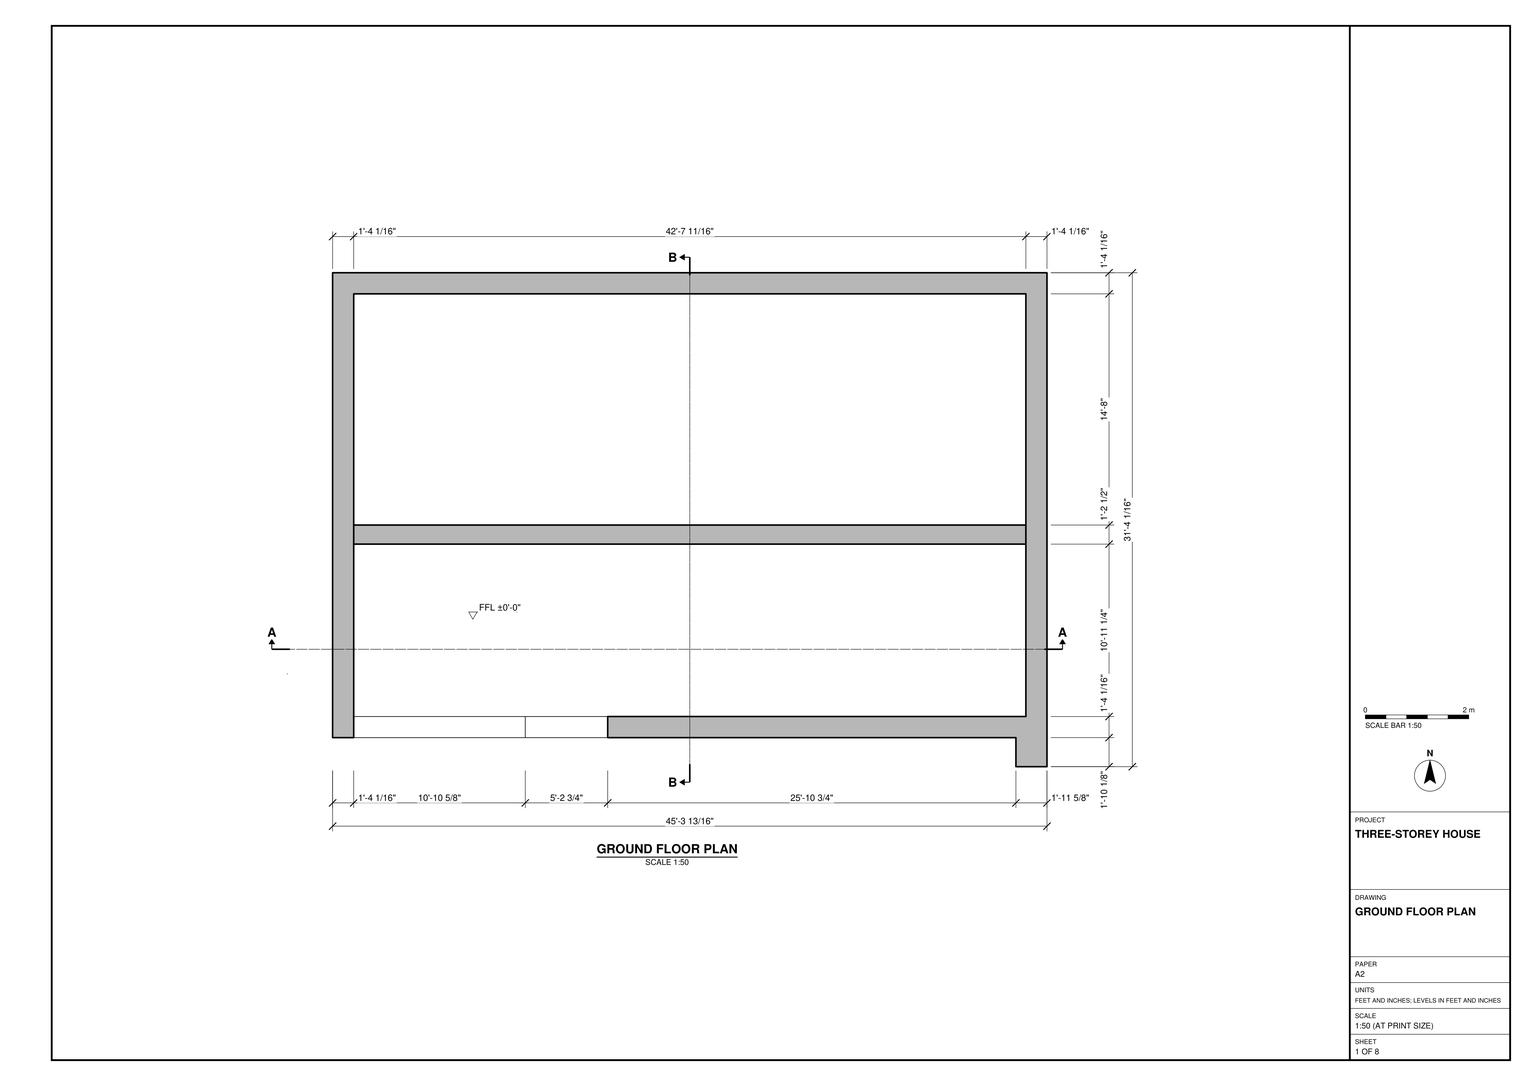
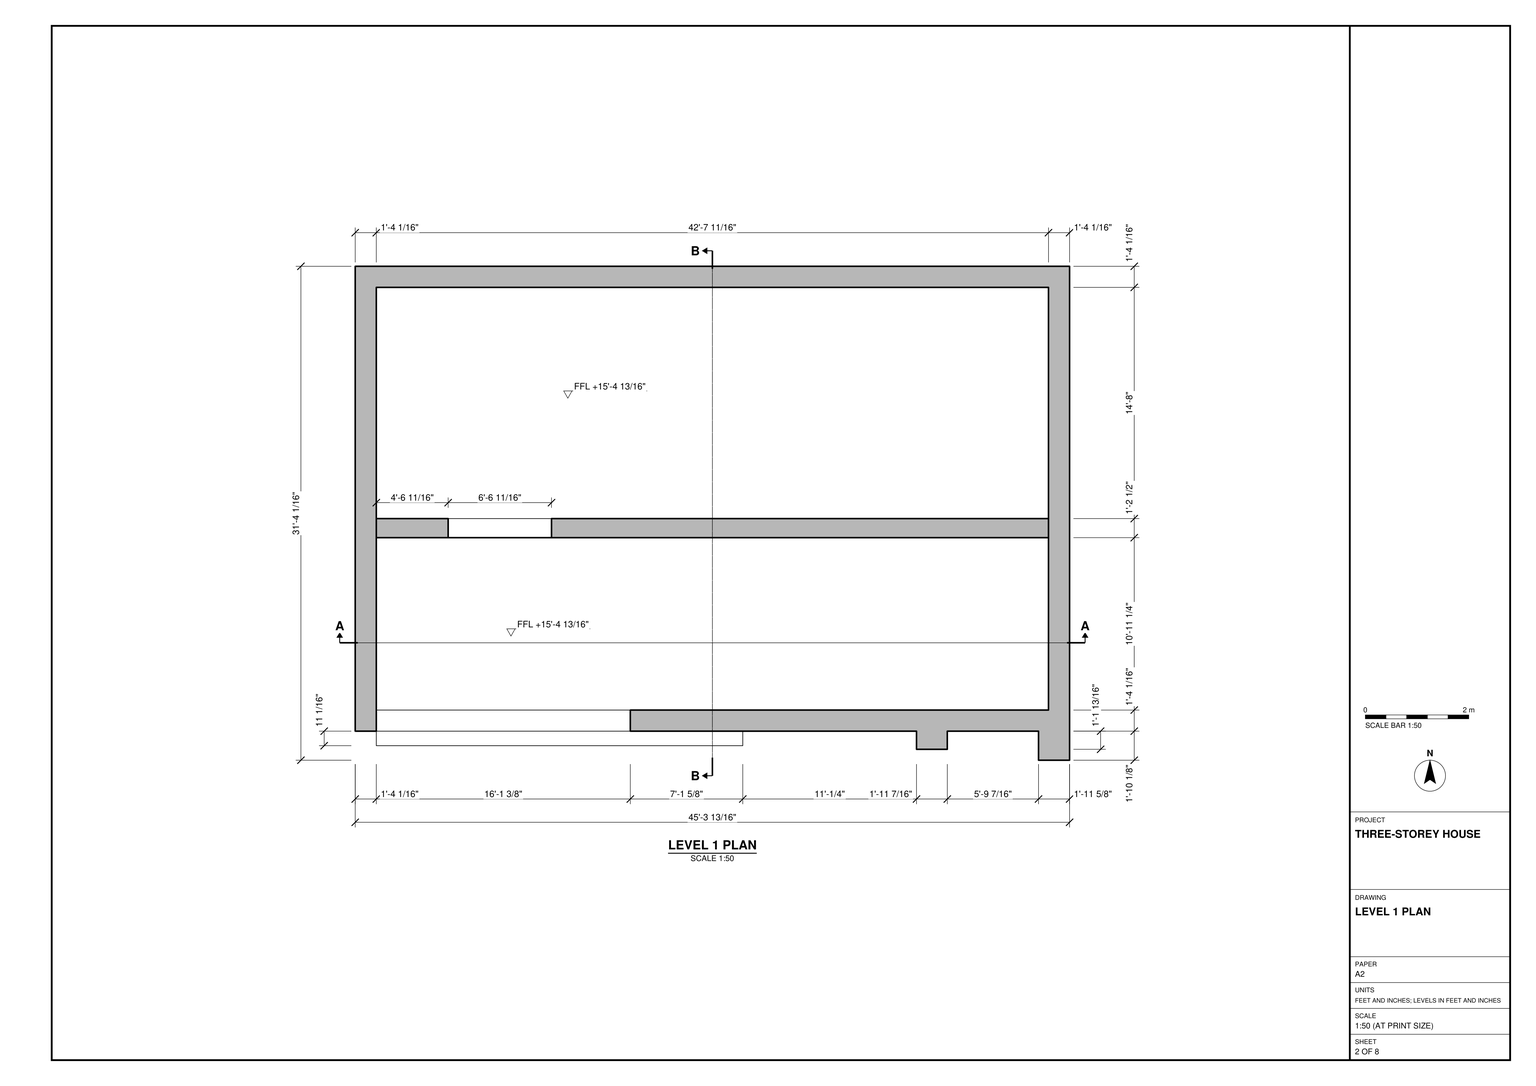
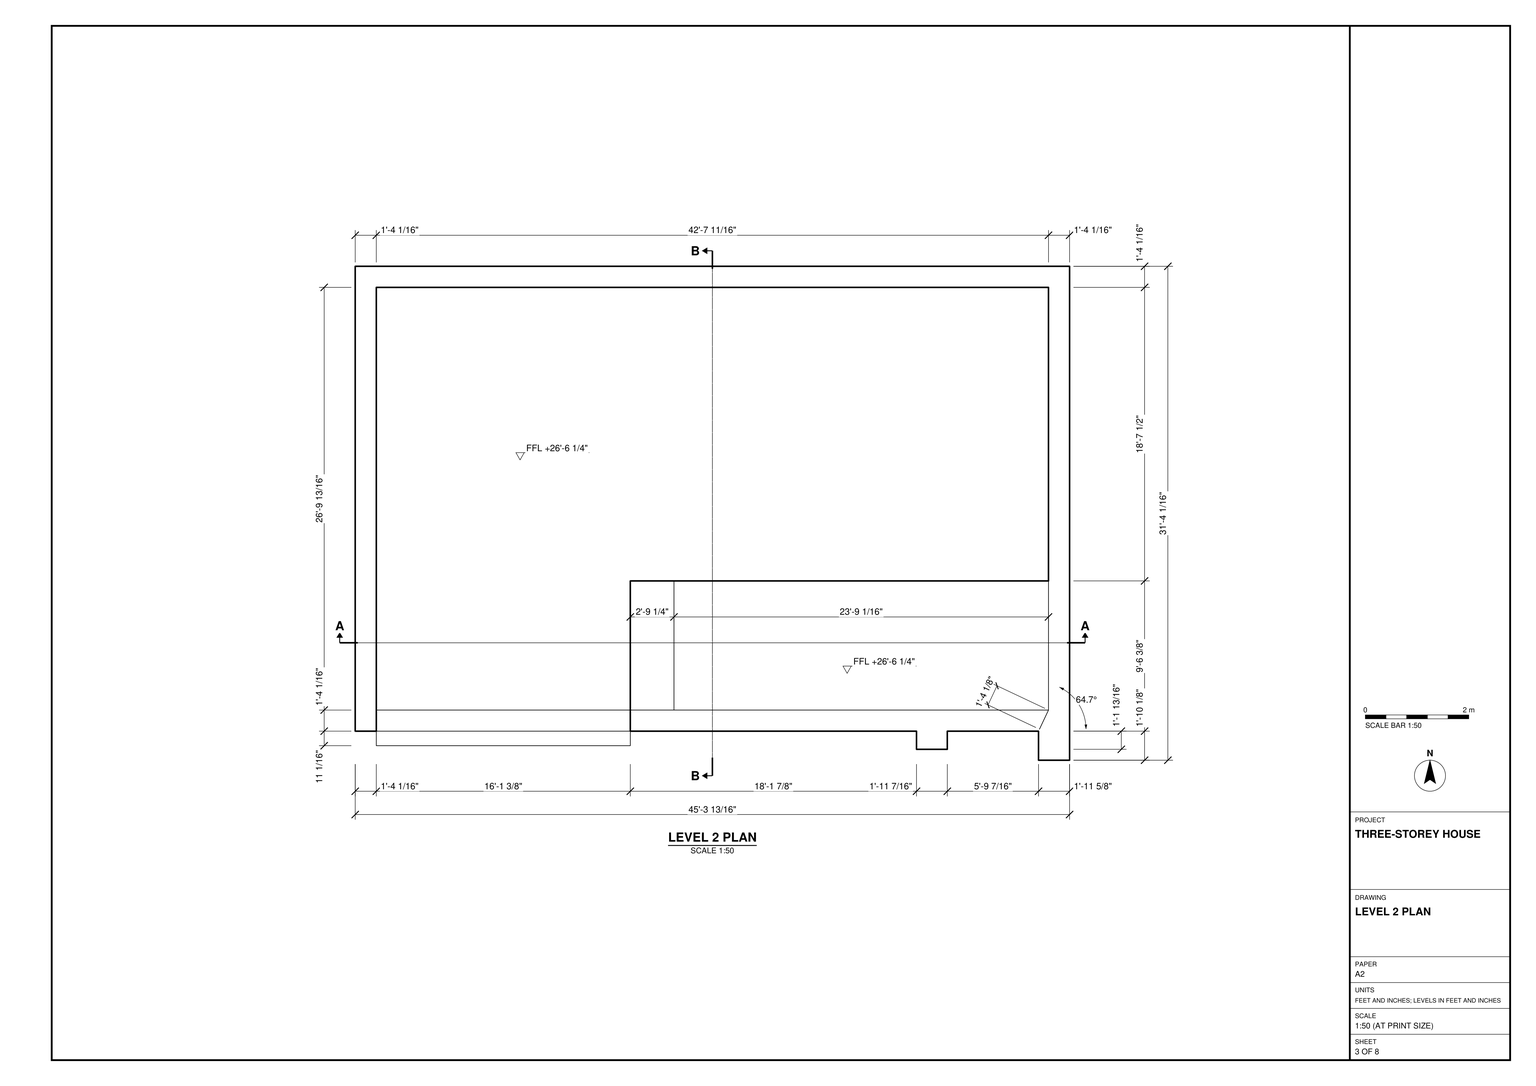
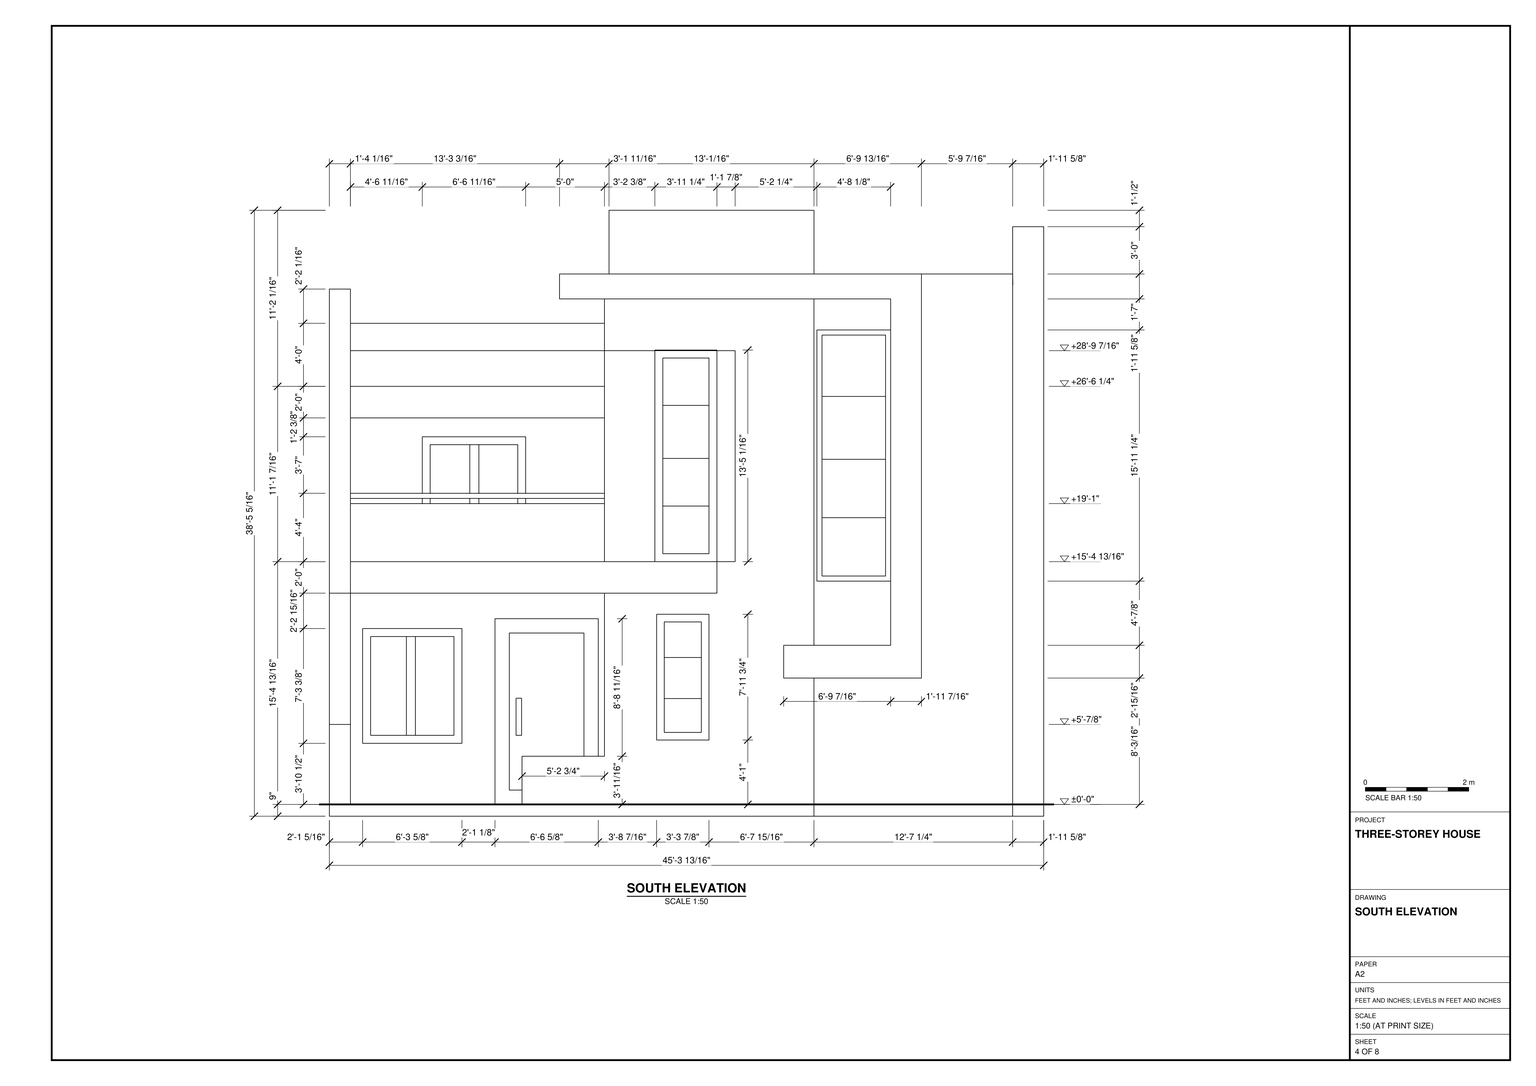
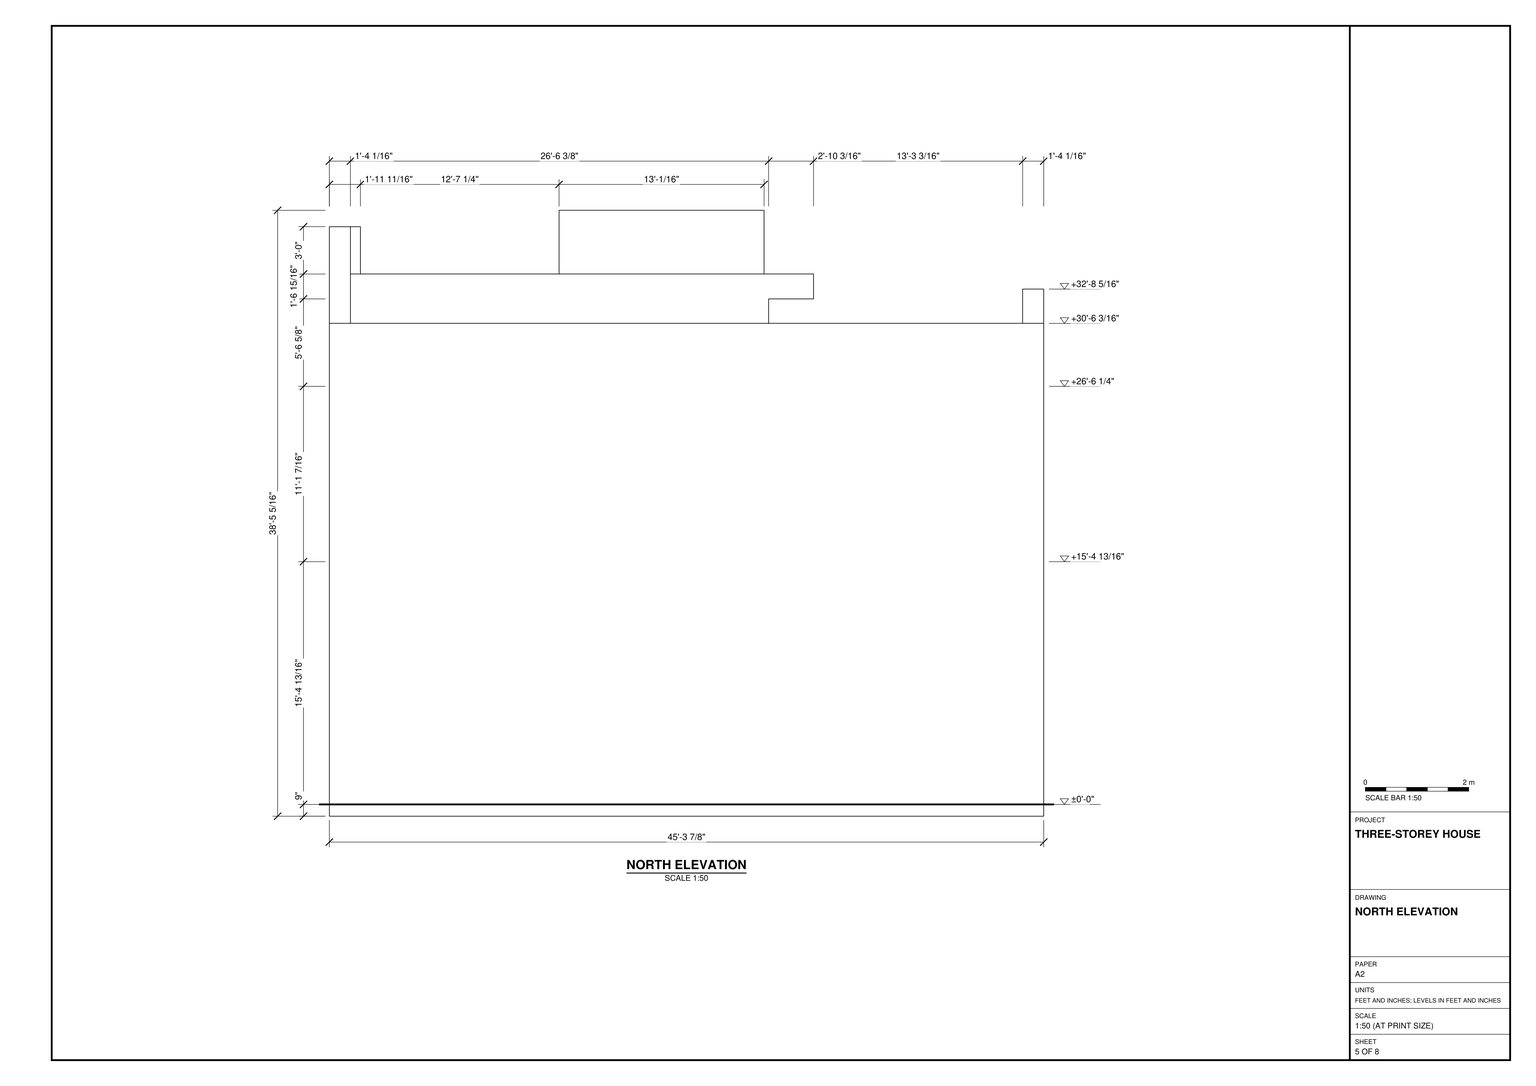
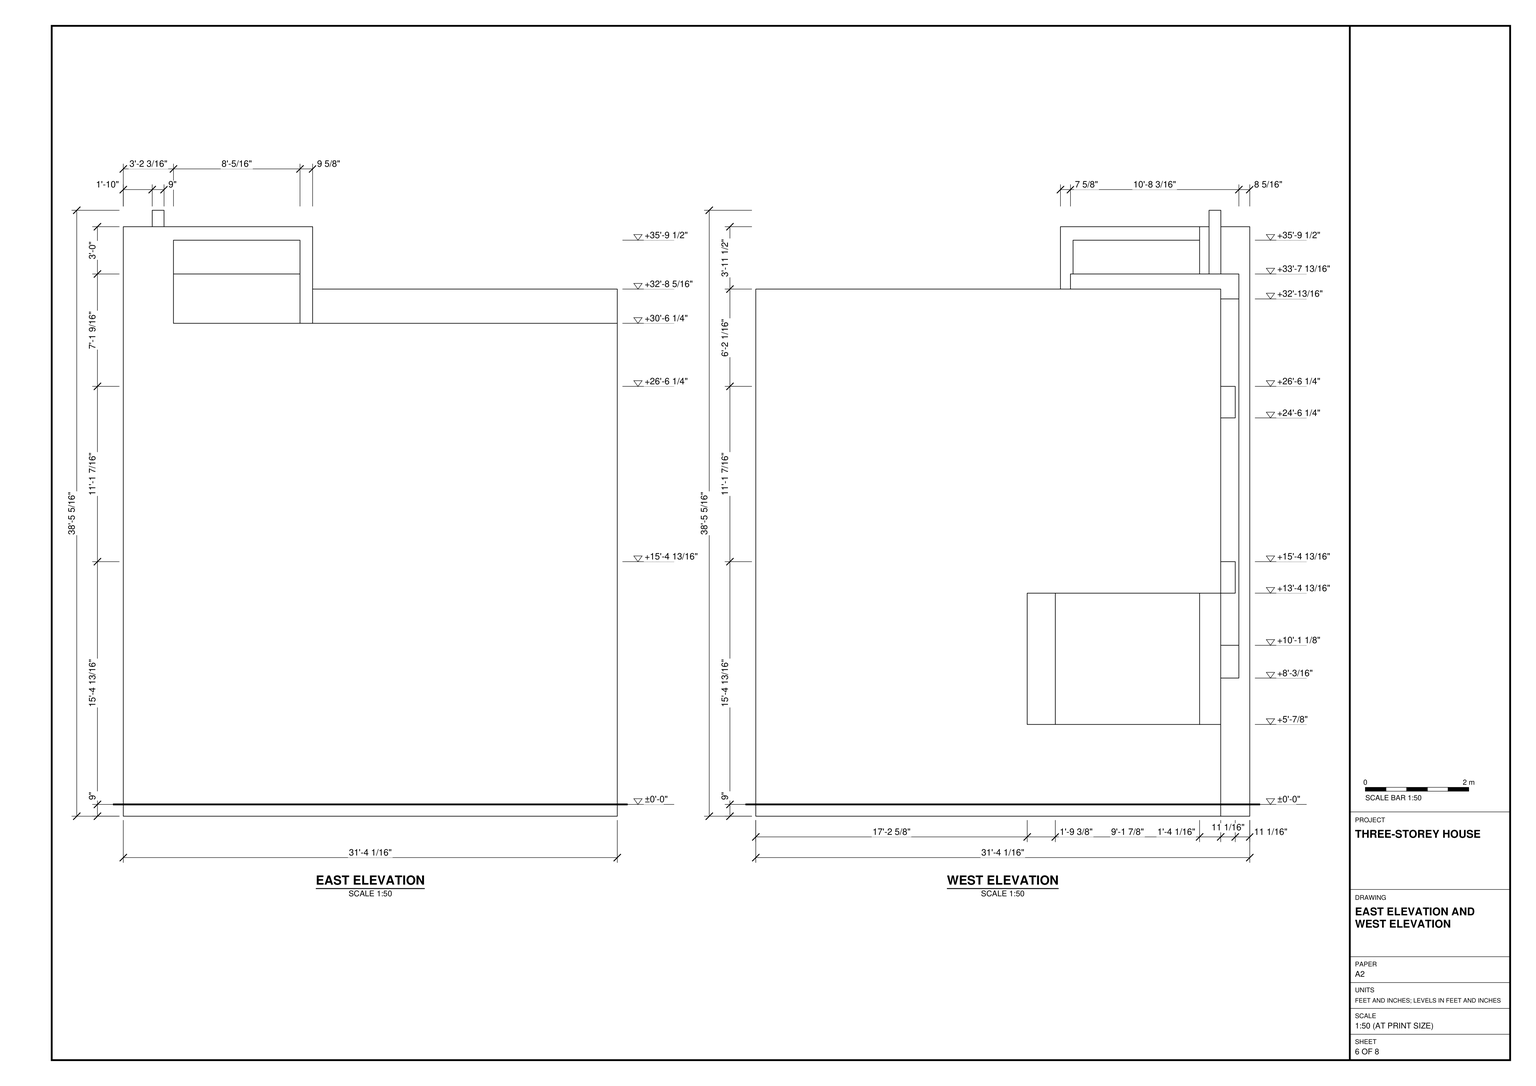
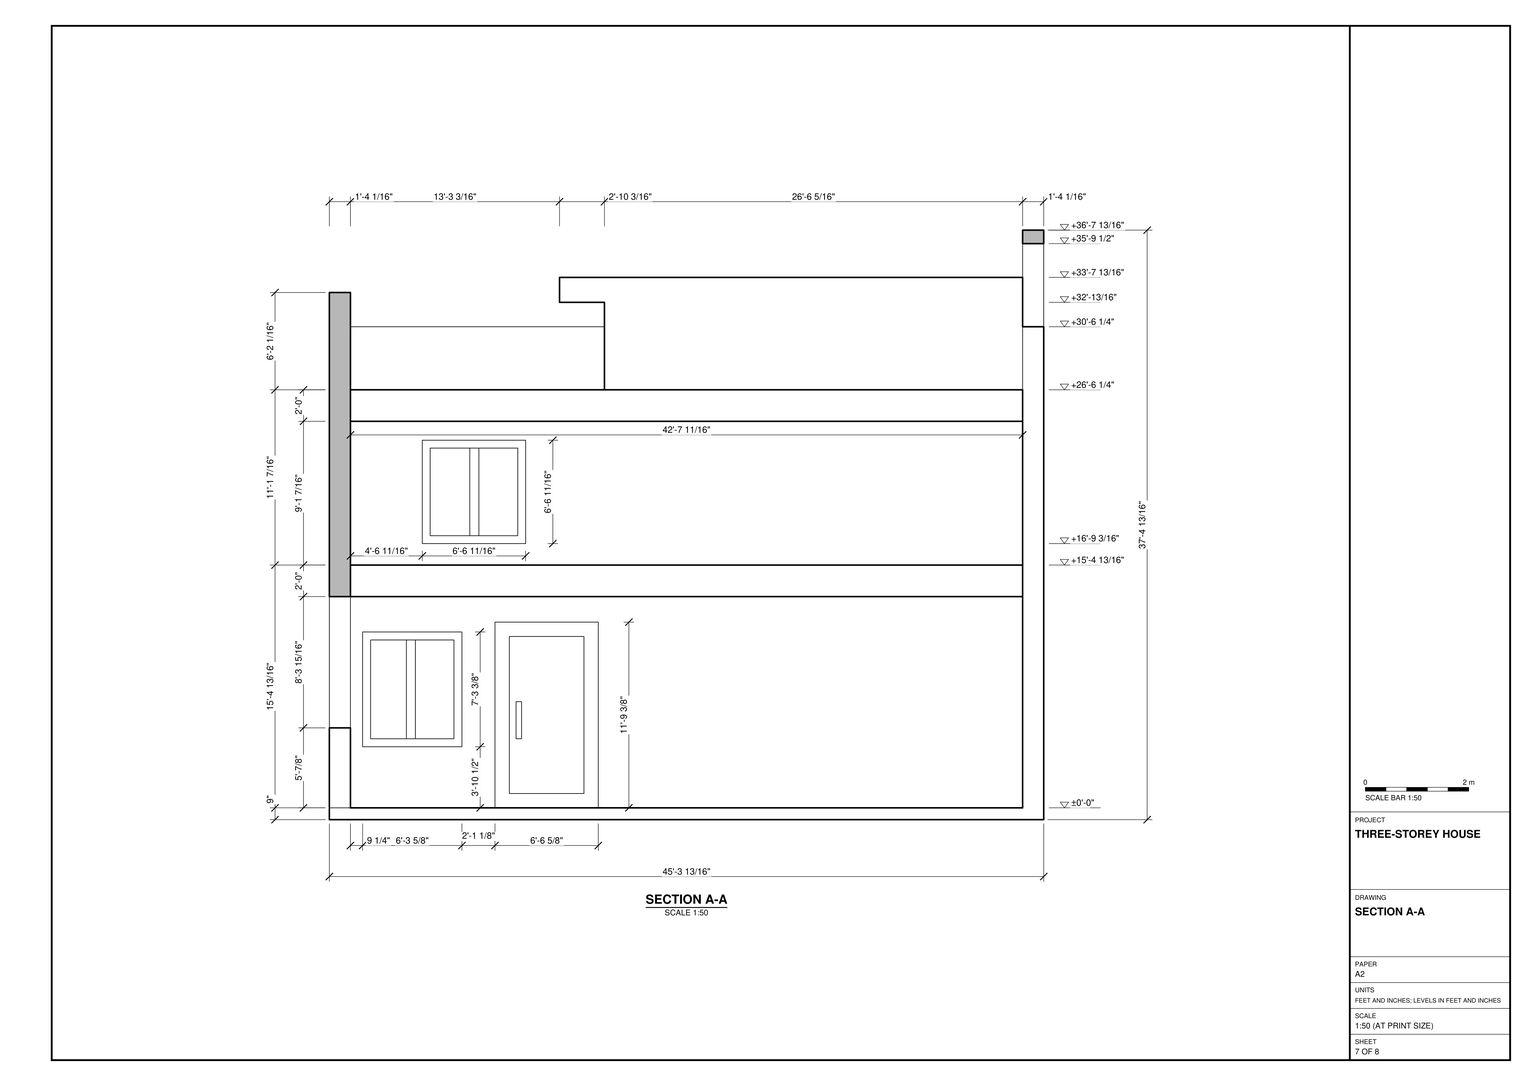
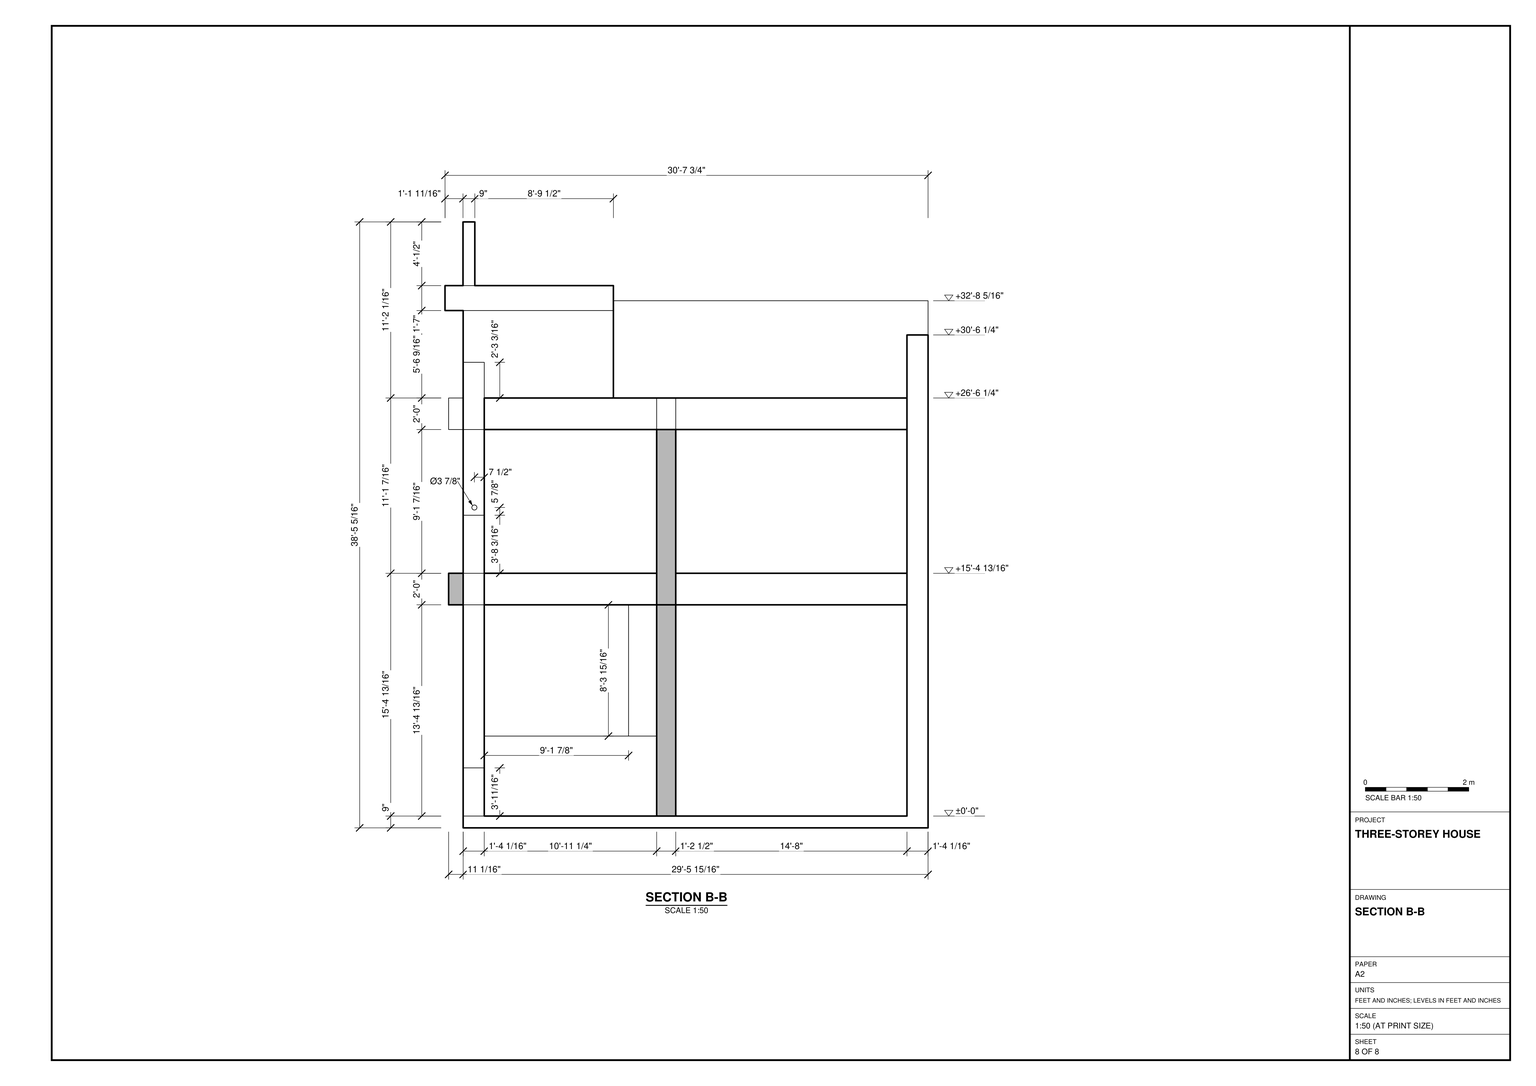
Build the three-storey house in SketchUp from task_files/diagram_01.pdf. Work in feet and inches. Set out the house with an overall east–west width of 45'-3 13/16", a north–south depth of 31'-4 1/16" and a height of 38'-5 5/16". Use finished floor levels of ±0'-0" for the ground floor, +15'-4 13/16" for Level 1 and +26'-6 1/4" for Level 2.

Use each storey's plan rather than copying the ground floor unchanged. On the two lower floors, build the perimeter walls and the east–west dividing wall to their drawn thicknesses. Keep the ground-floor dividing wall continuous, but form the opening near its west end on Level 1. Reproduce the broad opening at the west end of the south frontage, the projecting wall ends and the change in outline at the southeast of Level 2. Match the slabs and roof to the sheets, and model stairs, door and window units, built-in joinery and main furniture only where shown. Any decor or loose items shown may use suitable library components.

Keep walls, slabs and roof as separate groups or components. Group each furniture or joinery piece separately and use components for repeated parts. Save one SketchUp model as output_files/three_storey_house_with_a_stepped_south_frontage.skp.

# SketchUp Ruby script. Lengths in inches.
U = 1.inch
M = Sketchup.active_model
def pt(a) = Geom::Point3d.new(a.map { |v| v * U })
def face(e, loops, mat)
  f = e.add_face(loops[0].map { |a| pt(a) })
  loops[1..].each { |l| e.add_face(l.map { |a| pt(a) }).erase! }
  f.material = f.back_material = mat if mat
  f
end
# faces: each face lists its corners as indices into pts; further lists are holes
def faces(e, pts, list, mat = nil) = list.each { |f| face(e, (f[0].is_a?(Array) ? f : [f]).map { |l| l.map { |i| pts[i] } }, mat) }
# xy, xz, yz: faces in a plane at the given z, y or x. An outline is a flat list of corners, or four numbers for a rectangle; further outlines are holes
def ring(l) = l.size == 4 ? [[l[0], l[1]], [l[2], l[1]], [l[2], l[3]], [l[0], l[3]]] : l.each_slice(2).to_a
def flat(e, list, mat, &to3) = list.each { |f| face(e, (f[0].is_a?(Array) ? f : [f]).map { |l| ring(l).map { |u, v| to3.(u, v) } }, mat) }
def xy(e, z, list, mat = nil) = flat(e, list, mat) { |x, y| [x, y, z] }
def xz(e, y, list, mat = nil) = flat(e, list, mat) { |x, z| [x, y, z] }
def yz(e, x, list, mat = nil) = flat(e, list, mat) { |y, z| [x, y, z] }
def lines(e, pts, list) = list.each { |a, b| e.add_line(pt(pts[a]), pt(pts[b])) }
# prism: a flat outline (further loops are holes) pulled along v
def prism(e, loops, v, mat = nil)
  f = face(e, loops, mat); d = Geom::Vector3d.new(v.map { |x| x * U })
  f.pushpull(f.normal.samedirection?(d) ? d.length : -d.length)
end
def box(e, o, s, mat = nil) = prism(e, [[o, [o[0] + s[0], o[1], o[2]], [o[0] + s[0], o[1] + s[1], o[2]], [o[0], o[1] + s[1], o[2]]]], [0, 0, s[2]], mat)
def at(x, y, z, deg = 0) = Geom::Transformation.translation(pt([x, y, z])) * Geom::Transformation.rotation(ORIGIN, Z_AXIS, deg.degrees)
def axes(o, x, y, z) = Geom::Transformation.new([*x, 0, *y, 0, *z, 0, *pt(o).to_a, 1])
def part(name) = M.definitions.add(name)
# library, detail: a bought-in or finely detailed component or shape, given as its bounding box
def library(name, o, s) = part(name).tap { |d| box(d.entities, o, s) }
def detail(e, o, s) = box(e.add_group.entities, o, s)
def put(e, d, t, mat = nil) = e.add_instance(d, t).tap { |i| i.material = mat if mat }
def group(e, t, mat = nil) = e.add_group.tap { |g| g.transformation = t; g.material = mat if mat }.entities
root = M.entities
M.materials.add("[Cladding Siding White]").color = [207, 207, 207]
M.materials.add("[Color C01]").color = [255, 229, 204]
M.materials.add("[Color M07]").color = [58, 58, 58]
M.materials.add("[Concrete Block 8x8 Gray]").color = [157, 158, 154]
M.materials.add("[Formica Laminate Light]1").color = [213, 189, 164]
M.materials.add("[Formica Laminate Light]2").color = [213, 189, 164]
M.materials.add("[Formica Speckled Grey]").color = [94, 105, 111]
M.materials.add("[Terrazzo Tile Light]").color = [219, 217, 210]
M.materials.add("[Translucent Glass Safety]").color = [204, 235, 244]
M.materials["[Translucent Glass Safety]"].alpha = 0.5
M.materials.add("[Wood Floor Dark]").color = [153, 94, 42]
M.materials.add("[Wood Floor Light]").color = [204, 176, 127]
M.materials.add("[Wood Floor]").color = [155, 105, 61]
M.materials.add("[Wood Veneer 01]").color = [120, 70, 37]
M.materials.add("[Wood Veneer 02]").color = [68, 46, 32]
xy(root,0,[[520.18,0,520.18,22.125,0,22.125,0,376.04,543.83,376.04,543.83,0]])
xy(root,9,[[16.0625,22.125,146.67,38.1875],[16.0625,38.1875,527.76,169.4375],[16.0625,169.4375,527.76,183.96],[16.0625,183.96,527.76,359.98]])
xy(root,45.68,[[146.67,22.125,209.42,38.1875]])
xy(root,69.875,[[0,22.125,16.0625,148.04],[0,148.04,16.0625,169.4375]])
xy(root,105.1875,[[345.85,8.3125,450.73,22.125]],"[Formica Speckled Grey]")
xy(root,130.125,[[345.85,8.3125,427.29,22.125]],"[Formica Speckled Grey]")
xy(root,169.8125,[[0,22.125,16.0625,148.04],[209.42,22.125,242.67,38.1875],[16.0625,169.4375,527.76,183.96],[16.0625,183.96,527.76,359.98]])
xy(root,169.8125,[[16.0625,11.0625,16.0625,169.4375,527.76,169.4375,527.76,38.1875,209.42,38.1875,209.42,22.125,295.04,22.125,295.04,11.0625]],"[Formica Speckled Grey]")
xy(root,193.8125,[[209.42,22.125,242.67,38.1875],[16.0625,38.1875,527.76,169.4375],[16.0625,183.96,527.76,359.98]])
xy(root,193.8125,[[16.0625,11.0625,295.04,22.125]],"[Formica Speckled Grey]")
xy(root,210.18,[[70.75,169.4375,149.44,183.96]])
xy(root,238,[[16.0625,22.125,209.42,38.1875]],"[Translucent Glass Safety]")
xy(root,288.86,[[70.75,169.4375,149.44,183.96]])
xy(root,303.25,[[16.0625,169.4375,527.76,183.96],[16.0625,183.96,527.76,359.98]])
xy(root,303.25,[[16.0625,11.0625,16.0625,169.4375,527.76,169.4375,527.76,38.1875,209.42,38.1875,209.42,11.0625]],"[Wood Floor]")
xy(root,327.25,[[16.0625,38.1875,209.42,38.1875,209.42,136.5,527.76,136.5,527.76,359.98,16.0625,359.98],[209.42,38.1875,242.67,136.5],[242.67,38.1875,527.76,136.5]])
xy(root,327.25,[[16.0625,11.0625,209.42,22.125]],"[Wood Floor]")
xy(root,354.4375,[[16.0625,22.125,209.42,38.1875]],"[Terrazzo Tile Light]")
xy(root,375.25,[[527.76,38.1875,543.83,134.53],[527.76,134.53,543.83,144.125]])
xy(root,375.25,[[527.76,144.125,543.83,144.125,543.83,376.04,16.0625,376.04,16.0625,359.98,527.76,359.98]],"[Terrazzo Tile Light]")
xy(root,393.84,[[273.45,11.84,272.2,12.01,271.04,12.49,270.05,13.25,269.28,14.25,268.8,15.41,268.64,16.66,268.8,17.9,269.28,19.0625,270.05,20.06,271.04,20.82,272.2,21.31,273.45,21.47,274.69,21.31,275.85,20.82,276.85,20.06,277.62,19.0625,278.1,17.9,278.26,16.66,278.1,15.41,277.62,14.25,276.85,13.25,275.85,12.49,274.69,12.01],[332.26,11.84,331.01,12.01,329.85,12.49,328.86,13.25,328.09,14.25,327.61,15.41,327.45,16.66,327.61,17.9,328.09,19.0625,328.86,20.06,329.85,20.82,331.01,21.31,332.26,21.47,333.51,21.31,334.67,20.82,335.66,20.06,336.43,19.0625,336.91,17.9,337.07,16.66,336.91,15.41,336.43,14.25,335.66,13.25,334.67,12.49,333.51,12.01],[190.96,23.23,189.91,23.37,188.93,23.77,188.08,24.42,187.4375,25.26,187.03,26.24,186.89,27.29,187.03,28.34,187.4375,29.32,188.08,30.16,188.93,30.81,189.91,31.21,190.96,31.35,192.01,31.21,192.99,30.81,193.83,30.16,194.47,29.32,194.88,28.34,195.02,27.29,194.88,26.24,194.47,25.26,193.83,24.42,192.99,23.77,192.01,23.37],[190.96,52.66,189.91,52.8,188.93,53.21,188.08,53.85,187.4375,54.7,187.03,55.68,186.89,56.73,187.03,57.78,187.4375,58.76,188.08,59.6,188.93,60.24,189.91,60.65,190.96,60.79,192.01,60.65,192.99,60.24,193.83,59.6,194.47,58.76,194.88,57.78,195.02,56.73,194.88,55.68,194.47,54.7,193.83,53.85,192.99,53.21,192.01,52.8],[190.96,84.48,189.91,84.62,188.93,85.02,188.08,85.67,187.4375,86.51,187.03,87.49,186.89,88.54,187.03,89.59,187.4375,90.57,188.08,91.41,188.93,92.06,189.91,92.46,190.96,92.6,192.01,92.46,192.99,92.06,193.83,91.41,194.47,90.57,194.88,89.59,195.02,88.54,194.88,87.49,194.47,86.51,193.83,85.67,192.99,85.02,192.01,84.62],
  [190.96,118.54,189.91,118.68,188.93,119.08,188.08,119.73,187.4375,120.57,187.03,121.55,186.89,122.6,187.03,123.65,187.4375,124.63,188.08,125.47,188.93,126.12,189.91,126.53,190.96,126.66,192.01,126.53,192.99,126.12,193.83,125.47,194.47,124.63,194.88,123.65,195.02,122.6,194.88,121.55,194.47,120.57,193.83,119.73,192.99,119.08,192.01,118.68]])
xy(root,393.84,[[[175.23,8.3125,209.42,136.5],[190.96,118.54,192.01,118.68,192.99,119.08,193.83,119.73,194.47,120.57,194.88,121.55,195.02,122.6,194.88,123.65,194.47,124.63,193.83,125.47,192.99,126.12,192.01,126.53,190.96,126.66,189.91,126.53,188.93,126.12,188.08,125.47,187.4375,124.63,187.03,123.65,186.89,122.6,187.03,121.55,187.4375,120.57,188.08,119.73,188.93,119.08,189.91,118.68],[190.96,84.48,192.01,84.62,192.99,85.02,193.83,85.67,194.47,86.51,194.88,87.49,195.02,88.54,194.88,89.59,194.47,90.57,193.83,91.41,192.99,92.06,192.01,92.46,190.96,92.6,189.91,92.46,188.93,92.06,188.08,91.41,187.4375,90.57,187.03,89.59,186.89,88.54,187.03,87.49,187.4375,86.51,188.08,85.67,188.93,85.02,189.91,84.62],[190.96,52.66,192.01,52.8,192.99,53.21,193.83,53.85,194.47,54.7,194.88,55.68,195.02,56.73,194.88,57.78,194.47,58.76,193.83,59.6,192.99,60.24,192.01,60.65,190.96,60.79,189.91,60.65,188.93,60.24,188.08,59.6,187.4375,58.76,187.03,57.78,186.89,56.73,187.03,55.68,187.4375,54.7,188.08,53.85,188.93,53.21,189.91,52.8],[190.96,23.23,192.01,23.37,192.99,23.77,193.83,24.42,194.47,25.26,194.88,26.24,195.02,27.29,194.88,28.34,194.47,29.32,193.83,30.16,192.99,30.81,192.01,31.21,190.96,31.35,189.91,31.21,188.93,30.81,188.08,30.16,187.4375,29.32,187.03,28.34,186.89,27.29,187.03,26.24,187.4375,25.26,188.08,24.42,188.93,23.77,189.91,23.37]],[[209.42,8.3125,427.29,22.125],[273.45,11.84,274.69,12.01,275.85,12.49,276.85,13.25,277.62,14.25,278.1,15.41,278.26,16.66,278.1,17.9,277.62,19.0625,276.85,20.06,275.85,20.82,274.69,21.31,273.45,21.47,272.2,21.31,271.04,20.82,270.05,20.06,269.28,19.0625,268.8,17.9,268.64,16.66,268.8,15.41,269.28,14.25,270.05,13.25,271.04,12.49,272.2,12.01],[332.26,11.84,333.51,12.01,334.67,12.49,335.66,13.25,336.43,14.25,336.91,15.41,337.07,16.66,336.91,17.9,336.43,19.0625,335.66,20.06,334.67,20.82,333.51,21.31,332.26,21.47,331.01,21.31,329.85,20.82,328.86,20.06,328.09,19.0625,327.61,17.9,327.45,16.66,327.61,15.41,328.09,14.25,328.86,13.25,329.85,12.49,331.01,12.01]]],"[Formica Speckled Grey]")
xy(root,401.3125,[[0,22.125,16.0625,376.04]],"[Terrazzo Tile Light]")
xy(root,412.8125,[[[175.23,8.3125,450.73,8.3125,450.73,22.125,520.18,22.125,520.18,136.5,175.23,136.5],[212.91,22.01,368.94,31.01]],[520.18,38.1875,527.76,136.5]],"[Formica Speckled Grey]")
xy(root,438.53,[[527.76,38.1875,543.83,134.53]])
xy(root,448.8125,[[520.18,0,543.83,0,543.83,144.125,527.76,144.125,527.76,38.1875,520.18,38.1875]])
xy(root,461.3125,[[212.91,22.01,368.94,31.01]],"[Concrete Block 8x8 Gray]")
xz(root,0,[[520.18,0,543.83,448.8125]])
xz(root,8.3125,[[345.85,105.1875,450.73,105.1875,450.73,412.8125,175.23,412.8125,175.23,393.84,427.29,393.84,427.29,130.125,345.85,130.125]],"[Formica Speckled Grey]")
xz(root,11.0625,[[16.0625,169.8125,295.04,193.8125]],"[Formica Speckled Grey]")
xz(root,11.0625,[[16.0625,303.25,209.42,327.25]],"[Wood Floor]")
xz(root,22.01,[[212.91,412.8125,368.94,461.3125]],"[Concrete Block 8x8 Gray]")
xz(root,22.125,[[0,169.8125,16.0625,401.3125],[242.67,169.8125,295.04,193.8125],[247.8,354.4375,295.04,354.9]])
xz(root,22.125,[[368.92,130.125,427.29,130.125,427.29,178.97,371.15,178.97,371.15,370.19,427.29,370.19,427.29,393.84,368.92,393.84]],"[Cladding Siding White]")
xz(root,22.125,[[254.96,63.83,283.18,89.59],[254.96,89.59,283.18,120.84],[254.96,120.84,283.18,147.92],[375.04,182.86,423.4,227.29],[253.85,199.86,289,236.125],
  [375.04,227.29,423.4,271.72],[253.85,236.125,289,272.39],[375.04,271.72,423.4,319.6],[253.85,272.39,289,312.76],[253.85,312.76,289,348.85],
  [375.04,319.6,423.4,366.3]],"[Color C01]")
xz(root,22.125,[[[0,0,368.92,0,368.92,105.1875,345.85,105.1875,345.85,130.125,368.92,130.125,368.92,393.84,209.42,393.84,209.42,354.4375,247.8,354.4375,247.8,354.9,295.04,354.9,295.04,354.4375,308.92,354.4375,308.92,193.8125,295.04,193.8125,295.04,169.8125,209.42,169.8125,209.42,45.68,146.67,45.68,146.67,9,16.0625,9,16.0625,69.875,0,69.875],[249.14,58.01,289,153.74]]],"[Concrete Block 8x8 Gray]")
xz(root,22.125,[[209.42,193.8125,247.8,354.4375],[295.04,193.8125,308.92,354.4375],[16.0625,327.25,209.42,354.4375]],"[Formica Laminate Light]1")
xz(root,22.125,[[16.0625,193.8125,209.42,238]],"[Translucent Glass Safety]")
xz(root,22.125,[[368.92,0,520.18,0,520.18,412.8125,450.73,412.8125,450.73,105.1875,368.92,105.1875]],"[Wood Floor Dark]")
xz(root,22.125,[[[249.14,58.01,289,153.74],[254.96,63.83,283.18,147.92]],[[371.15,178.97,427.29,370.19],[375.04,182.86,423.4,366.3]],[[247.8,193.8125,295.04,354.4375],[253.85,199.86,289,348.85]]],"[Wood Veneer 01]")
xz(root,31.01,[[212.91,412.8125,368.94,461.3125]],"[Concrete Block 8x8 Gray]")
xz(root,38.1875,[[146.67,9,146.67,45.68,209.42,45.68,209.42,169.8125,527.76,169.8125,527.76,9],[242.67,169.8125,527.76,193.8125],[209.42,193.8125,527.76,303.25],[209.42,303.25,242.67,327.25],[242.67,303.25,527.76,327.25],
  [16.0625,327.25,209.42,354.4375],[527.76,375.25,543.83,438.53],[520.18,412.8125,527.76,448.8125]])
xz(root,38.1875,[[16.0625,193.8125,209.42,238]],"[Translucent Glass Safety]")
xz(root,134.53,[[527.76,375.25,543.83,438.53]])
xz(root,136.5,[[209.42,327.25,209.42,393.84,175.23,393.84,175.23,412.8125,527.76,412.8125,527.76,327.25]],"[Formica Speckled Grey]")
xz(root,144.125,[[527.76,375.25,543.83,448.8125]])
xz(root,148.04,[[0,69.875,16.0625,169.8125]])
xz(root,169.4375,[[0,69.875,16.0625,169.8125],[16.0625,169.8125,527.76,193.8125]])
xz(root,169.4375,[[31.41,61.59,58.65,136.8],[65.51,61.59,94.86,136.8],[76.75,216.17,106.91,282.87],[113.84,216.17,143.45,282.87]],"[Color C01]")
xz(root,169.4375,[[[16.0625,9,126.1,9,126.1,150.375,204.72,150.375,204.72,9,527.76,9,527.76,169.8125,16.0625,169.8125],[25.32,55.51,100.94,142.88]],[[16.0625,193.8125,527.76,303.25],[70.75,210.18,149.44,288.86]]],"[Formica Laminate Light]1")
xz(root,169.4375,[[142.14,61.59,146.34,89.85]],"[Wood Floor Light]")
xz(root,169.4375,[[[126.1,9,204.72,150.375],[137,19.91,193.8125,139.47]],[[137,19.91,193.8125,139.47],[142.14,61.59,146.34,89.85]],[[25.32,55.51,100.94,142.88],[31.41,61.59,94.86,136.8]],[58.65,61.59,65.51,136.8],[[70.75,210.18,149.44,288.86],[76.75,216.17,143.45,282.87]],
  [106.91,216.17,113.84,282.87]],"[Wood Veneer 02]")
xz(root,183.96,[[16.0625,9,527.76,169.8125],[16.0625,169.8125,527.76,193.8125],[[16.0625,193.8125,527.76,303.25],[70.75,210.18,149.44,288.86]]])
xz(root,359.98,[[16.0625,9,527.76,169.8125],[16.0625,169.8125,527.76,193.8125],[16.0625,193.8125,527.76,303.25],[16.0625,303.25,527.76,327.25],[16.0625,327.25,527.76,375.25]])
xz(root,376.04,[[0,0,543.83,375.25],[0,375.25,16.0625,401.3125]],"[Terrazzo Tile Light]")
yz(root,0,[[148.04,69.875,169.4375,169.8125]])
yz(root,0,[[22.125,0,22.125,69.875,169.4375,69.875,169.4375,169.8125,22.125,169.8125,22.125,401.3125,376.04,401.3125,376.04,0]],"[Terrazzo Tile Light]")
yz(root,16.0625,[[22.125,9,38.1875,69.875],[169.4375,9,183.96,169.8125],[183.96,9,359.98,169.8125],[22.125,169.8125,169.4375,169.8125,169.4375,193.8125,38.1875,193.8125,38.1875,238,22.125,238],[169.4375,169.8125,183.96,303.25],
  [183.96,169.8125,359.98,193.8125],[183.96,193.8125,359.98,303.25],[22.125,303.25,38.1875,354.4375],[38.1875,303.25,169.4375,327.25],[169.4375,303.25,183.96,327.25],
  [183.96,303.25,359.98,327.25],[38.1875,327.25,359.98,327.25,359.98,375.25,376.04,375.25,376.04,401.3125,22.125,401.3125,22.125,354.4375,38.1875,354.4375]])
yz(root,16.0625,[[38.1875,9,169.4375,69.875],[148.04,69.875,169.4375,169.8125],[[38.1875,193.8125,169.4375,193.8125,169.4375,303.25,22.125,303.25,22.125,238,38.1875,238],[30.67,241.96,30.17,242.02,29.7,242.22,29.3,242.53,28.99,242.93,28.8,243.39,28.73,243.9,28.8,244.4,28.99,244.86,29.3,245.27,29.7,245.57,30.17,245.77,30.67,245.83,31.17,245.77,31.64,245.57,32.04,245.27,32.35,244.86,32.54,244.4,32.61,243.9,32.54,243.39,32.35,242.93,32.04,242.53,31.64,242.22,31.17,242.02]]],"[Formica Laminate Light]1")
yz(root,16.0625,[[11.0625,169.8125,22.125,193.8125]],"[Formica Speckled Grey]")
yz(root,16.0625,[[11.0625,303.25,22.125,327.25]],"[Wood Floor]")
yz(root,70.75,[[169.4375,210.18,183.96,288.86]])
yz(root,146.67,[[22.125,9,38.1875,45.68]])
yz(root,149.44,[[169.4375,210.18,183.96,288.86]])
yz(root,175.23,[[8.3125,393.84,136.5,412.8125]],"[Formica Speckled Grey]")
yz(root,209.42,[[22.125,45.68,38.1875,169.8125],[22.125,193.8125,38.1875,238],[30.67,241.96,31.17,242.02,31.64,242.22,32.04,242.53,32.35,242.93,32.54,243.39,32.61,243.9,32.54,244.4,32.35,244.86,32.04,245.27,31.64,245.57,31.17,245.77,30.67,245.83,30.17,245.77,29.7,245.57,29.3,245.27,28.99,244.86,28.8,244.4,28.73,243.9,28.8,243.39,28.99,242.93,29.3,242.53,29.7,242.22,30.17,242.02],[22.125,303.25,38.1875,354.4375]])
yz(root,209.42,[[[22.125,238,38.1875,303.25],[30.67,241.96,31.17,242.02,31.64,242.22,32.04,242.53,32.35,242.93,32.54,243.39,32.61,243.9,32.54,244.4,32.35,244.86,32.04,245.27,31.64,245.57,31.17,245.77,30.67,245.83,30.17,245.77,29.7,245.57,29.3,245.27,28.99,244.86,28.8,244.4,28.73,243.9,28.8,243.39,28.99,242.93,29.3,242.53,29.7,242.22,30.17,242.02]]],"[Formica Laminate Light]2")
yz(root,209.42,[[38.1875,327.25,38.1875,354.4375,22.125,354.4375,22.125,393.84,136.5,393.84,136.5,327.25]],"[Formica Speckled Grey]")
yz(root,209.42,[[11.0625,303.25,22.125,327.25]],"[Wood Floor]")
yz(root,212.91,[[22.01,412.8125,31.01,461.3125]],"[Concrete Block 8x8 Gray]")
yz(root,242.67,[[22.125,169.8125,38.1875,193.8125]])
yz(root,295.04,[[11.0625,169.8125,22.125,193.8125]],"[Formica Speckled Grey]")
yz(root,345.85,[[8.3125,105.1875,22.125,130.125]],"[Formica Speckled Grey]")
yz(root,368.94,[[22.01,412.8125,31.01,461.3125]],"[Concrete Block 8x8 Gray]")
yz(root,427.29,[[8.3125,130.125,22.125,393.84]],"[Formica Speckled Grey]")
yz(root,450.73,[[8.3125,105.1875,22.125,412.8125]],"[Formica Speckled Grey]")
yz(root,520.18,[[0,0,0,448.8125,38.1875,448.8125,38.1875,412.8125,22.125,412.8125,22.125,0]])
yz(root,527.76,[[169.4375,9,183.96,169.8125],[183.96,9,359.98,169.8125],[38.1875,169.8125,169.4375,193.8125],[169.4375,169.8125,183.96,303.25],[183.96,169.8125,359.98,193.8125],
  [183.96,193.8125,359.98,303.25],[38.1875,303.25,169.4375,327.25],[169.4375,303.25,183.96,327.25],[183.96,303.25,359.98,327.25],[136.5,327.25,169.4375,375.25],
  [169.4375,327.25,183.96,375.25],[183.96,327.25,359.98,375.25],[136.5,375.25,136.5,412.8125,134.53,412.8125,134.53,438.53,38.1875,438.53,38.1875,448.8125,144.125,448.8125,144.125,375.25],[134.53,375.25,136.5,412.8125]])
yz(root,527.76,[[38.1875,9,169.4375,169.8125],[38.1875,193.8125,169.4375,303.25]],"[Formica Laminate Light]1")
yz(root,527.76,[[38.1875,375.25,134.53,412.8125]],"[Formica Speckled Grey]")
yz(root,543.83,[[[0,0,376.04,0,376.04,375.25,144.125,375.25,144.125,448.8125,0,448.8125],[38.1875,375.25,134.53,438.53]]],"[Terrazzo Tile Light]")
p = [[209.42,30.17,242.02],[209.42,29.7,242.22],[16.0625,29.7,242.22],[16.0625,30.17,242.02],[209.42,30.67,241.96],[16.0625,30.67,241.96],
  [209.42,31.17,242.02],[16.0625,31.17,242.02],[209.42,31.64,242.22],[16.0625,31.64,242.22],[209.42,29.3,242.53],[16.0625,29.3,242.53],
  [209.42,32.04,242.53],[16.0625,32.04,242.53],[209.42,28.99,242.93],[16.0625,28.99,242.93],[209.42,32.35,242.93],[16.0625,32.35,242.93],
  [209.42,28.8,243.39],[16.0625,28.8,243.39],[209.42,32.54,243.39],[16.0625,32.54,243.39],[209.42,28.73,243.9],[16.0625,28.73,243.9],
  [209.42,32.61,243.9],[16.0625,32.61,243.9],[209.42,28.8,244.4],[16.0625,28.8,244.4],[209.42,32.54,244.4],[16.0625,32.54,244.4],
  [209.42,28.99,244.86],[16.0625,28.99,244.86],[209.42,32.35,244.86],[16.0625,32.35,244.86],[209.42,29.3,245.27],[16.0625,29.3,245.27],
  [209.42,32.04,245.27],[16.0625,32.04,245.27],[209.42,29.7,245.57],[16.0625,29.7,245.57],[209.42,31.64,245.57],[16.0625,31.64,245.57],
  [209.42,30.17,245.77],[16.0625,30.17,245.77],[209.42,31.17,245.77],[16.0625,31.17,245.77],[209.42,30.67,245.83],[16.0625,30.67,245.83],
  [-34.49,70.43,0],[-34.49,70.9375,0],[0,169.4375,9],[16.0625,169.4375,9],[527.76,38.1875,0],[527.76,38.1875,9],
  [520.18,22.125,412.8125]]
faces(root,p,[[0,1,2,3],[4,0,3,5],[6,4,5,7],[8,6,7,9],[1,10,11,2],[12,8,9,13],[10,14,15,11],[16,12,13,17],
  [14,18,19,15],[20,16,17,21],[18,22,23,19],[24,20,21,25],[22,26,27,23],[28,24,25,29],[26,30,31,27],[32,28,29,33],
  [30,34,35,31],[36,32,33,37],[34,38,39,35],[40,36,37,41],[38,42,43,39],[44,40,41,45],[42,46,47,43],[46,44,45,47]],"[Color M07]")
lines(root,p,[[48,49],[50,51],[52,53],[54,52]])
